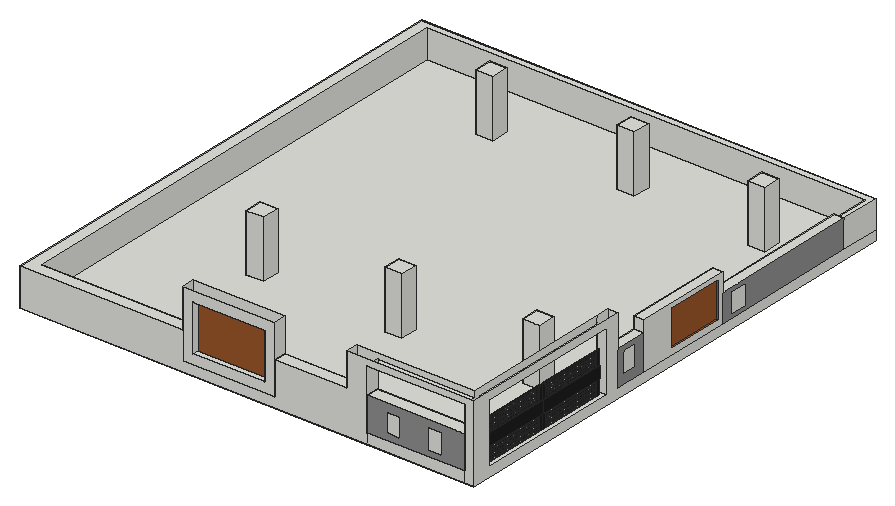
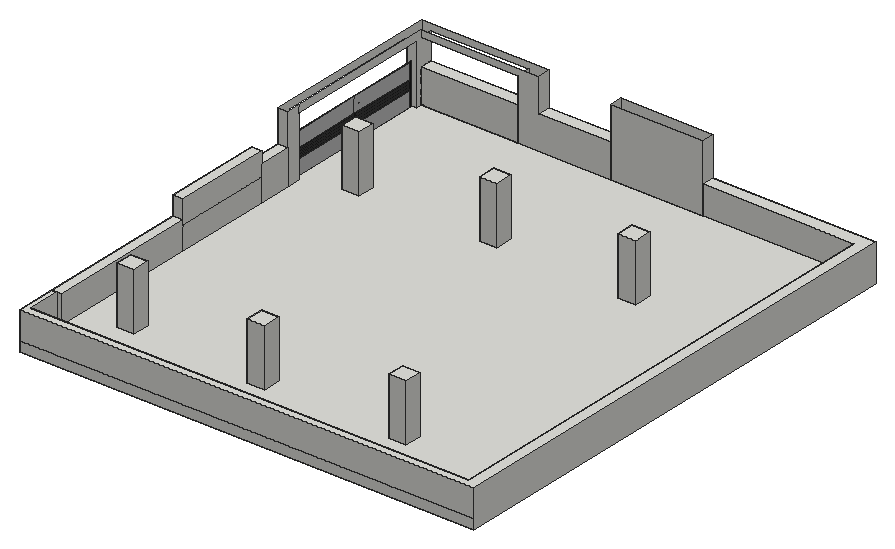
# SketchUp Ruby script. Lengths in inches.
U = 1.inch
M = Sketchup.active_model
def pt(a) = Geom::Point3d.new(a.map { |v| v * U })
def face(e, loops, mat)
  f = e.add_face(loops[0].map { |a| pt(a) })
  loops[1..].each { |l| e.add_face(l.map { |a| pt(a) }).erase! }
  f.material = f.back_material = mat if mat
  f
end
# faces: each face lists its corners as indices into pts; further lists are holes
def faces(e, pts, list, mat = nil) = list.each { |f| face(e, (f[0].is_a?(Array) ? f : [f]).map { |l| l.map { |i| pts[i] } }, mat) }
# xy, xz, yz: faces in a plane at the given z, y or x. An outline is a flat list of corners, or four numbers for a rectangle; further outlines are holes
def ring(l) = l.size == 4 ? [[l[0], l[1]], [l[2], l[1]], [l[2], l[3]], [l[0], l[3]]] : l.each_slice(2).to_a
def flat(e, list, mat, &to3) = list.each { |f| face(e, (f[0].is_a?(Array) ? f : [f]).map { |l| ring(l).map { |u, v| to3.(u, v) } }, mat) }
def xy(e, z, list, mat = nil) = flat(e, list, mat) { |x, y| [x, y, z] }
def xz(e, y, list, mat = nil) = flat(e, list, mat) { |x, z| [x, y, z] }
def yz(e, x, list, mat = nil) = flat(e, list, mat) { |y, z| [x, y, z] }
def lines(e, pts, list) = list.each { |a, b| e.add_line(pt(pts[a]), pt(pts[b])) }
# prism: a flat outline (further loops are holes) pulled along v
def prism(e, loops, v, mat = nil)
  f = face(e, loops, mat); d = Geom::Vector3d.new(v.map { |x| x * U })
  f.pushpull(f.normal.samedirection?(d) ? d.length : -d.length)
end
def box(e, o, s, mat = nil) = prism(e, [[o, [o[0] + s[0], o[1], o[2]], [o[0] + s[0], o[1] + s[1], o[2]], [o[0], o[1] + s[1], o[2]]]], [0, 0, s[2]], mat)
def at(x, y, z, deg = 0) = Geom::Transformation.translation(pt([x, y, z])) * Geom::Transformation.rotation(ORIGIN, Z_AXIS, deg.degrees)
def axes(o, x, y, z) = Geom::Transformation.new([*x, 0, *y, 0, *z, 0, *pt(o).to_a, 1])
def part(name) = M.definitions.add(name)
# library, detail: a bought-in or finely detailed component or shape, given as its bounding box
def library(name, o, s) = part(name).tap { |d| box(d.entities, o, s) }
def detail(e, o, s) = box(e.add_group.entities, o, s)
def put(e, d, t, mat = nil) = e.add_instance(d, t).tap { |i| i.material = mat if mat }
def group(e, t, mat = nil) = e.add_group.tap { |g| g.transformation = t; g.material = mat if mat }.entities
root = M.entities
M.materials.add("Color_008").color = [30, 30, 30]
M.materials.add("[0055_LightGoldenrodYellow]").color = [250, 250, 210]
M.materials.add("[0131_Silver]").color = [192, 192, 192]
M.materials.add("[0134_DimGray]").color = [105, 105, 105]
M.materials.add("[Color M04]").color = [142, 142, 142]
M.materials.add("[Wood Cherry Original]").color = [152, 86, 42]
c1 = part("Gate infill panel")
box(c1.entities,[0,0,-9.84],[39.64,0.39,36.58])
c2 = part("Gate frame upright")
box(c2.entities,[0,0,0],[1.9,0.97,93.54])
c3 = part("Square gate bar")
box(c3.entities,[2.95,0,-2.03],[0.99,0.97,40.94])
c4 = part("Rectangular gate slat")
box(c4.entities,[0,0,-2.03],[1.97,0.97,40.94])
c5 = part("Slatted gate panel")
p = [[42.85,0.97,43.31],[42.85,0.97,44.29]]
lines(c5.entities,p,[[0,1]])
put(c5.entities,c2,axes([87.6,0,0],[1,0,0],[0,1,0],[0,0,0.92593]),"Color_008")
put(c5.entities,c2,axes([0,0,0],[1,0,0],[0,1,0],[0,0,0.92593]),"Color_008")
put(c5.entities,c2,axes([42.85,0,0],[1,0,0],[0,1,0],[0,0,0.92593]),"Color_008")
put(c5.entities,c2,axes([44.75,0,0],[1,0,0],[0,1,0],[0,0,0.92593]),"Color_008")
put(c5.entities,c3,axes([3.9375,0,6.89],[0,0,-1],[0,1,0],[1,0,0]),"[0134_DimGray]")
put(c5.entities,c3,axes([48.6875,0,6.89],[0,0,-1],[0,1,0],[1,0,0]),"[0134_DimGray]")
put(c5.entities,c3,axes([48.6875,0,11.71],[0,0,-1],[0,1,0],[1,0,0]),"[0134_DimGray]")
put(c5.entities,c4,axes([48.6875,0,6.79],[0,0,-1],[0,1,0],[1,0,0]),"Color_008")
put(c5.entities,c4,axes([3.9375,0,6.79],[0,0,-1],[0,1,0],[1,0,0]),"Color_008")
put(c5.entities,c3,axes([3.9375,0,11.71],[0,0,-1],[0,1,0],[1,0,0]),"[0134_DimGray]")
put(c5.entities,c4,axes([3.9375,0,11.61],[0,0,-1],[0,1,0],[1,0,0]),"Color_008")
put(c5.entities,c3,axes([3.9375,0,16.54],[0,0,-1],[0,1,0],[1,0,0]),"[0134_DimGray]")
put(c5.entities,c3,axes([48.6875,0,16.54],[0,0,-1],[0,1,0],[1,0,0]),"[0134_DimGray]")
put(c5.entities,c3,axes([48.6875,0,21.36],[0,0,-1],[0,1,0],[1,0,0]),"[0134_DimGray]")
put(c5.entities,c4,axes([48.6875,0,11.61],[0,0,-1],[0,1,0],[1,0,0]),"Color_008")
put(c5.entities,c3,axes([3.9375,0,21.36],[0,0,-1],[0,1,0],[1,0,0]),"[0134_DimGray]")
put(c5.entities,c4,axes([3.9375,0,26.08],[0,0,-1],[0,1,0],[1,0,0]),"Color_008")
put(c5.entities,c3,axes([3.9375,0,31],[0,0,-1],[0,1,0],[1,0,0]),"[0134_DimGray]")
put(c5.entities,c3,axes([3.9375,0,26.18],[0,0,-1],[0,1,0],[1,0,0]),"[0134_DimGray]")
put(c5.entities,c4,axes([48.6875,0,30.91],[0,0,-1],[0,1,0],[1,0,0]),"Color_008")
put(c5.entities,c4,axes([48.6875,0,21.26],[0,0,-1],[0,1,0],[1,0,0]),"Color_008")
put(c5.entities,c4,axes([3.9375,0,21.26],[0,0,-1],[0,1,0],[1,0,0]),"Color_008")
put(c5.entities,c4,axes([48.6875,0,41.7],[0,0,-1],[0,1,0],[1,0,0]),"Color_008")
put(c5.entities,c4,axes([48.6875,0,26.08],[0,0,-1],[0,1,0],[1,0,0]),"Color_008")
put(c5.entities,c4,axes([3.9375,0,35.73],[0,0,-1],[0,1,0],[1,0,0]),"Color_008")
put(c5.entities,c4,axes([3.9375,0,41.7],[0,0,-1],[0,1,0],[1,0,0]),"Color_008")
put(c5.entities,c4,axes([48.6875,0,35.73],[0,0,-1],[0,1,0],[1,0,0]),"Color_008")
put(c5.entities,c3,axes([48.6875,0,31],[0,0,-1],[0,1,0],[1,0,0]),"[0134_DimGray]")
put(c5.entities,c3,axes([48.6875,0,26.18],[0,0,-1],[0,1,0],[1,0,0]),"[0134_DimGray]")
put(c5.entities,c3,axes([3.9375,0,67.42],[0,0,-1],[0,1,0],[1,0,0]),"[0134_DimGray]")
put(c5.entities,c4,axes([48.6875,0,57.68],[0,0,-1],[0,1,0],[1,0,0]),"Color_008")
put(c5.entities,c4,axes([48.6875,0,52.85],[0,0,-1],[0,1,0],[1,0,0]),"Color_008")
put(c5.entities,c4,axes([3.9375,0,30.91],[0,0,-1],[0,1,0],[1,0,0]),"Color_008")
put(c5.entities,c3,axes([48.6875,0,57.78],[0,0,-1],[0,1,0],[1,0,0]),"[0134_DimGray]")
put(c5.entities,c4,axes([48.6875,0,62.5],[0,0,-1],[0,1,0],[1,0,0]),"Color_008")
put(c5.entities,c4,axes([3.9375,0,57.68],[0,0,-1],[0,1,0],[1,0,0]),"Color_008")
put(c5.entities,c4,axes([3.9375,0,62.5],[0,0,-1],[0,1,0],[1,0,0]),"Color_008")
put(c5.entities,c3,axes([48.6875,0,67.42],[0,0,-1],[0,1,0],[1,0,0]),"[0134_DimGray]")
put(c5.entities,c3,axes([48.6875,0,62.6],[0,0,-1],[0,1,0],[1,0,0]),"[0134_DimGray]")
put(c5.entities,c3,axes([3.9375,0,62.6],[0,0,-1],[0,1,0],[1,0,0]),"[0134_DimGray]")
put(c5.entities,c4,axes([48.6875,0,46.88],[0,0,-1],[0,1,0],[1,0,0]),"Color_008")
put(c5.entities,c4,axes([3.9375,0,52.85],[0,0,-1],[0,1,0],[1,0,0]),"Color_008")
put(c5.entities,c4,axes([3.9375,0,46.88],[0,0,-1],[0,1,0],[1,0,0]),"Color_008")
put(c5.entities,c3,axes([3.9375,0,57.78],[0,0,-1],[0,1,0],[1,0,0]),"[0134_DimGray]")
put(c5.entities,c4,axes([48.6875,0,16.4375],[0,0,-1],[0,1,0],[1,0,0]),"Color_008")
put(c5.entities,c4,axes([3.9375,0,16.4375],[0,0,-1],[0,1,0],[1,0,0]),"Color_008")
put(c5.entities,c4,axes([48.6875,0,1.97],[0,0,-1],[0,1,0],[1,0,0]),"Color_008")
put(c5.entities,c4,axes([3.9375,0,1.97],[0,0,-1],[0,1,0],[1,0,0]),"Color_008")
put(c5.entities,c3,axes([3.9375,0,81.89],[0,0,-1],[0,1,0],[1,0,0]),"[0134_DimGray]")
put(c5.entities,c4,axes([48.6875,0,72.15],[0,0,-1],[0,1,0],[1,0,0]),"Color_008")
put(c5.entities,c4,axes([48.6875,0,67.32],[0,0,-1],[0,1,0],[1,0,0]),"Color_008")
put(c5.entities,c3,axes([48.6875,0,72.24],[0,0,-1],[0,1,0],[1,0,0]),"[0134_DimGray]")
put(c5.entities,c3,axes([3.9375,0,72.24],[0,0,-1],[0,1,0],[1,0,0]),"[0134_DimGray]")
put(c5.entities,c4,axes([3.9375,0,72.15],[0,0,-1],[0,1,0],[1,0,0]),"Color_008")
put(c5.entities,c3,axes([3.9375,0,77.07],[0,0,-1],[0,1,0],[1,0,0]),"[0134_DimGray]")
put(c5.entities,c3,axes([48.6875,0,81.89],[0,0,-1],[0,1,0],[1,0,0]),"[0134_DimGray]")
put(c5.entities,c4,axes([3.9375,0,76.97],[0,0,-1],[0,1,0],[1,0,0]),"Color_008")
put(c5.entities,c4,axes([48.6875,0,76.97],[0,0,-1],[0,1,0],[1,0,0]),"Color_008")
put(c5.entities,c3,axes([48.6875,0,77.07],[0,0,-1],[0,1,0],[1,0,0]),"[0134_DimGray]")
put(c5.entities,c4,axes([3.9375,0,67.32],[0,0,-1],[0,1,0],[1,0,0]),"Color_008")
put(c5.entities,c4,axes([48.6875,0,86.61],[0,0,-1],[0,1,0],[1,0,0]),"Color_008")
put(c5.entities,c4,axes([48.6875,0,81.79],[0,0,-1],[0,1,0],[1,0,0]),"Color_008")
put(c5.entities,c3,axes([3.9375,0,86.71],[0,0,-1],[0,1,0],[1,0,0]),"[0134_DimGray]")
put(c5.entities,c3,axes([48.6875,0,86.71],[0,0,-1],[0,1,0],[1,0,0]),"[0134_DimGray]")
put(c5.entities,c4,axes([3.9375,0,86.61],[0,0,-1],[0,1,0],[1,0,0]),"Color_008")
put(c5.entities,c4,axes([3.9375,0,81.79],[0,0,-1],[0,1,0],[1,0,0]),"Color_008")
put(c5.entities,c3,axes([48.6875,0,35.83],[0,0,-1],[0,1,0],[1,0,0]),"[0134_DimGray]")
put(c5.entities,c3,axes([3.9375,0,35.83],[0,0,-1],[0,1,0],[1,0,0]),"[0134_DimGray]")
c6 = part("Gate infill panel \#1")
box(c6.entities,[0,0,-1.97],[52.81,0.39,23.62])
c7 = part("Porton casa")
put(c7.entities,c1,axes([268.93,-49.21,9.91],[1.04618,0,0],[0,1,0],[0,0,0.8072]),"[0131_Silver]")
put(c7.entities,c1,axes([227.46,-49.21,63.0625],[1.04618,0,0],[0,1,0],[0,0,0.8072]),"[0131_Silver]")
put(c7.entities,c5,axes([225.62,-50.18,0],[0.96774,0,0],[0,1,0],[0,0,1]),"[0055_LightGoldenrodYellow]")
put(c7.entities,c1,axes([227.46,-49.21,9.91],[1.04618,0,0],[0,1,0],[0,0,0.8072]),"[0131_Silver]")
put(c7.entities,c6,axes([225.62,-50.57,33.46],[0.82011,0,0],[0,1,0],[0,0,1]),"Color_008")
put(c7.entities,c1,axes([268.93,-49.21,63.0625],[1.04618,0,0],[0,1,0],[0,0,0.8072]),"[0131_Silver]")
put(c7.entities,c6,axes([268.93,-50.57,33.46],[0.82011,0,0],[0,1,0],[0,0,1]),"Color_008")
c8 = part("Group\#88")
box(c8.entities,[0,0,0],[36.75,36.75,120])
xy(root,18.77,[[0,0,950.48,1049.5625]])
xy(root,39.08,[[340.16,0,532.72,27.4375],[24.125,26.71,340.16,26.71,340.16,27.4375,929.91,27.4375,929.91,38.75,950.48,38.75,950.48,345.07,929.91,345.07,929.91,966.48,939.96,966.48,939.96,1034.92,24.125,1034.92],[929.91,374.76,950.48,443.45],[929.91,443.45,950.48,648.82],[929.91,648.82,950.48,966.48]])
xy(root,40.08,[[725.85,0,929.91,27.4375]])
xy(root,50.27,[[945.41,514.35,950.48,638.33]],"[Wood Cherry Original]")
xy(root,60.1875,[[361.27,0,511.62,13.4375]])
xy(root,97.39,[[0,0,340.16,0,340.16,26.71,24.125,26.71,24.125,1034.92,939.96,1034.92,939.96,966.48,950.48,966.48,950.48,1049.5625,0,1049.5625],[929.91,648.82,950.48,966.48]])
xy(root,109.08,[[532.72,0,683.66,27.4375]])
xy(root,110.64,[[725.85,0,929.91,27.4375]])
xy(root,112.04,[[929.91,374.76,950.48,443.45]])
xy(root,126.89,[[945.41,514.35,950.48,638.33]],"[Wood Cherry Original]")
xy(root,136.6,[[929.91,443.45,950.48,648.82]])
xy(root,157.98,[[361.27,0,511.62,13.4375]])
xz(root,0,[[0,18.77,725.85,18.77,725.85,166.08,929.91,166.08,929.91,18.77,950.48,18.77,950.48,179.08,683.66,179.08,683.66,109.08,532.72,109.08,532.72,39.08,340.16,39.08,340.16,97.39,0,97.39],[725.85,18.77,929.91,40.08],[[340.16,39.08,532.72,179.08],[361.27,60.1875,511.62,157.98]],[855.78,53.87,880.97,94.63],[767.07,53.95,795.51,94.76]])
xz(root,0,[[[725.85,40.08,929.91,110.64],[767.07,53.95,795.51,94.76],[855.78,53.87,880.97,94.63]]],"[Color M04]")
xz(root,13.4375,[[361.27,60.1875,511.62,157.98]],"[Wood Cherry Original]")
xz(root,26.71,[[24.125,39.08,340.16,97.39]])
xz(root,27.4375,[[340.16,39.08,532.72,179.08],[532.72,39.08,532.72,109.08,683.66,109.08,683.66,179.08,929.91,179.08,929.91,166.08,725.85,166.08,725.85,39.08],[725.85,39.08,929.91,40.08],[725.85,40.08,929.91,110.64]])
xz(root,38.75,[[929.91,39.08,950.48,163.67]])
xz(root,345.07,[[929.91,39.08,950.48,163.67]])
xz(root,374.76,[[929.91,39.08,950.48,112.04],[929.91,112.04,950.48,179.08]])
xz(root,443.45,[[929.91,39.08,950.48,112.04],[929.91,112.04,950.48,136.6]])
xz(root,514.35,[[945.41,50.27,950.48,126.89]],"[Wood Cherry Original]")
xz(root,638.33,[[945.41,50.27,950.48,126.89]],"[Wood Cherry Original]")
xz(root,648.82,[[929.91,39.08,950.48,97.39],[929.91,97.39,950.48,136.6]])
xz(root,966.48,[[929.91,39.08,939.96,97.39],[939.96,39.08,950.48,97.39]])
xz(root,1034.92,[[24.125,39.08,939.96,97.39]])
xz(root,1049.5625,[[0,18.77,950.48,39.08],[0,39.08,950.48,97.39]])
yz(root,0,[[0,18.77,1049.5625,97.39]])
yz(root,24.125,[[26.71,39.08,1034.92,97.39]])
yz(root,340.16,[[26.71,39.08,26.71,97.39,0,97.39,0,179.08,27.4375,179.08,27.4375,39.08]])
yz(root,361.27,[[0,60.1875,13.4375,157.98]])
yz(root,511.62,[[0,60.1875,13.4375,109.08],[0,109.08,13.4375,157.98]])
yz(root,532.72,[[0,39.08,27.4375,109.08],[0,109.08,27.4375,179.08]])
yz(root,683.66,[[0,109.08,27.4375,179.08]])
yz(root,725.85,[[0,40.08,27.4375,110.64],[0,110.64,27.4375,166.08]])
yz(root,929.91,[[27.4375,39.08,27.4375,110.64,0,110.64,0,166.08,27.4375,166.08,27.4375,179.08,345.07,179.08,345.07,163.67,38.75,163.67,38.75,39.08],[345.07,39.08,374.76,179.08],[374.76,39.08,443.45,112.04],[443.45,39.08,648.82,86.85],[648.82,39.08,966.48,97.39],
  [0,40.08,27.4375,110.64],[443.45,86.85,648.82,136.6]])
yz(root,939.96,[[966.48,39.08,1034.92,97.39]])
yz(root,945.41,[[514.35,50.27,638.33,126.89]],"[Wood Cherry Original]")
yz(root,950.48,[[[0,18.77,1049.5625,18.77,1049.5625,39.08,374.76,39.08,374.76,179.08,0,179.08],[38.75,39.08,345.07,163.67]],[[443.45,39.08,648.82,136.6],[514.35,50.27,638.33,126.89]],[966.48,39.08,1049.5625,97.39],[669.87,45.75,709.12,88.4375],[390.47,60.2,415.85,101.26]])
yz(root,950.48,[[[374.76,39.08,443.45,112.04],[390.47,60.2,415.85,101.26]],[[648.82,39.08,966.48,97.39],[669.87,45.75,709.12,88.4375]]],"[Color M04]")
put(root,c7,axes([890.33,-737.13,37.11],[0,3.4472,0],[-1,0,0],[0,0,1]))
put(root,c8,axes([855.6,879.04,159.08],[-1,0,0],[0,1,0],[0,0,-1]))
put(root,c8,axes([855.6,290.67,159.08],[-1,0,0],[0,1,0],[0,0,-1]))
put(root,c8,axes([277.6,290.67,159.08],[-1,0,0],[0,1,0],[0,0,-1]))
put(root,c8,axes([277.6,890.4,159.08],[-1,0,0],[0,1,0],[0,0,-1]))
put(root,c8,axes([572.73,890.4,159.08],[-1,0,0],[0,1,0],[0,0,-1]))
put(root,c8,axes([572.73,283.65,159.08],[-1,0,0],[0,1,0],[0,0,-1]))
